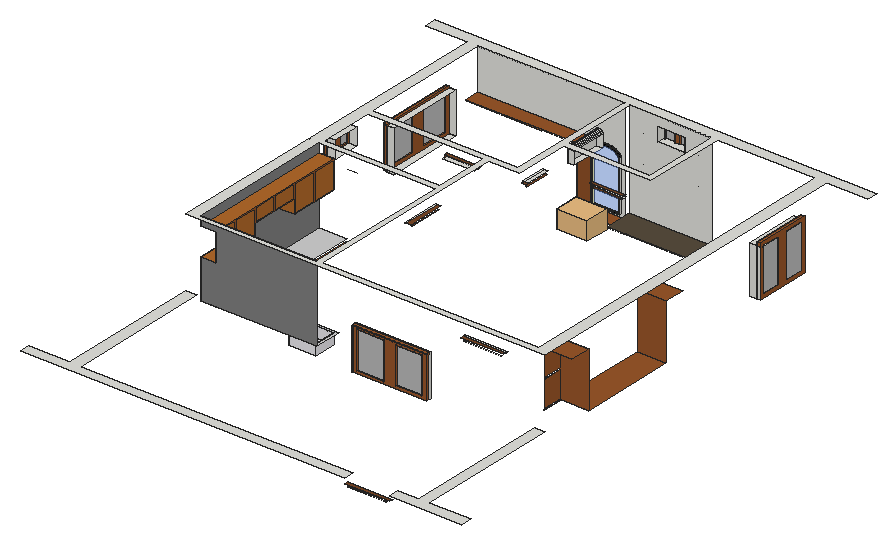
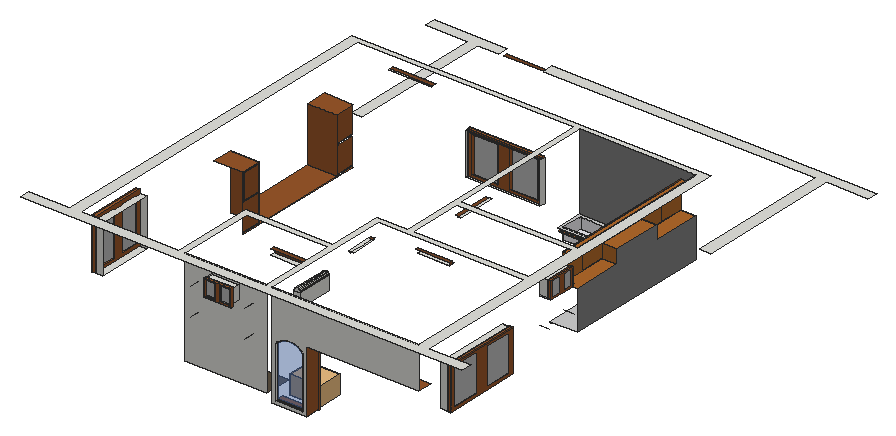
# SketchUp Ruby script. Lengths in inches.
U = 1.inch
M = Sketchup.active_model
def pt(a) = Geom::Point3d.new(a.map { |v| v * U })
def face(e, loops, mat)
  f = e.add_face(loops[0].map { |a| pt(a) })
  loops[1..].each { |l| e.add_face(l.map { |a| pt(a) }).erase! }
  f.material = f.back_material = mat if mat
  f
end
# faces: each face lists its corners as indices into pts; further lists are holes
def faces(e, pts, list, mat = nil) = list.each { |f| face(e, (f[0].is_a?(Array) ? f : [f]).map { |l| l.map { |i| pts[i] } }, mat) }
# xy, xz, yz: faces in a plane at the given z, y or x. An outline is a flat list of corners, or four numbers for a rectangle; further outlines are holes
def ring(l) = l.size == 4 ? [[l[0], l[1]], [l[2], l[1]], [l[2], l[3]], [l[0], l[3]]] : l.each_slice(2).to_a
def flat(e, list, mat, &to3) = list.each { |f| face(e, (f[0].is_a?(Array) ? f : [f]).map { |l| ring(l).map { |u, v| to3.(u, v) } }, mat) }
def xy(e, z, list, mat = nil) = flat(e, list, mat) { |x, y| [x, y, z] }
def xz(e, y, list, mat = nil) = flat(e, list, mat) { |x, z| [x, y, z] }
def yz(e, x, list, mat = nil) = flat(e, list, mat) { |y, z| [x, y, z] }
def lines(e, pts, list) = list.each { |a, b| e.add_line(pt(pts[a]), pt(pts[b])) }
# prism: a flat outline (further loops are holes) pulled along v
def prism(e, loops, v, mat = nil)
  f = face(e, loops, mat); d = Geom::Vector3d.new(v.map { |x| x * U })
  f.pushpull(f.normal.samedirection?(d) ? d.length : -d.length)
end
def box(e, o, s, mat = nil) = prism(e, [[o, [o[0] + s[0], o[1], o[2]], [o[0] + s[0], o[1] + s[1], o[2]], [o[0], o[1] + s[1], o[2]]]], [0, 0, s[2]], mat)
def at(x, y, z, deg = 0) = Geom::Transformation.translation(pt([x, y, z])) * Geom::Transformation.rotation(ORIGIN, Z_AXIS, deg.degrees)
def axes(o, x, y, z) = Geom::Transformation.new([*x, 0, *y, 0, *z, 0, *pt(o).to_a, 1])
def part(name) = M.definitions.add(name)
# library, detail: a bought-in or finely detailed component or shape, given as its bounding box
def library(name, o, s) = part(name).tap { |d| box(d.entities, o, s) }
def detail(e, o, s) = box(e.add_group.entities, o, s)
def put(e, d, t, mat = nil) = e.add_instance(d, t).tap { |i| i.material = mat if mat }
def group(e, t, mat = nil) = e.add_group.tap { |g| g.transformation = t; g.material = mat if mat }.entities
root = M.entities
M.materials.add("[0133_Gray]").color = [128, 128, 128]
M.materials.add("[Carpet Diamond Olive]").color = [87, 77, 61]
M.materials.add("[Carrera Marble]").color = [207, 207, 207]
M.materials.add("[Color E01]").color = [255, 255, 204]
M.materials.add("[Color M09]").color = [0, 0, 0]
M.materials.add("[Metal Silver]").color = [234, 233, 238]
M.materials.add("[Mirror 01]").color = [185, 185, 185]
M.materials.add("[Translucent Glass Blue]").color = [100, 149, 237]
M.materials["[Translucent Glass Blue]"].alpha = 0.5
M.materials.add("[Wood Bamboo]").color = [177, 105, 43]
M.materials.add("[Wood Cherry Original]").color = [152, 86, 42]
M.materials.add("[Wood Veneer 01]").color = [120, 70, 37]
xy(root,40.7,[[157.82,411.42,158.26,411.48,158.67,411.64,159.02,411.87,159.28,412.16,159.43,412.49,159.47,412.85,159.39,413.2,159.19,413.52,158.9,413.79,158.53,413.99,158.1,414.11,157.65,414.14,157.21,414.08,156.8,413.93,156.45,413.7,156.2,413.41,156.04,413.07,156,412.72,156.08,412.37,156.28,412.05,156.57,411.77,156.94,411.57,157.37,411.45]])
xy(root,41.76,[[142.67,429.03,172.1875,429.09]],"[Wood Cherry Original]")
xy(root,42,[[142.43,429.03,172.43,441.09]],"[Wood Cherry Original]")
xy(root,44.5,[[145.43,439.34,169.43,441.09]],"[Color M09]")
xy(root,45.45,[[146.38,439.34,168.48,439.84]],"[Color E01]")
xy(root,47.48,[[177.45,416.84,191.41,417.09]],"[Wood Cherry Original]")
xy(root,47.52,[[234.125,416.84,248.17,417.09]],"[Wood Cherry Original]")
xy(root,47.61,[[192.32,416.84,233.26,417.09]],"[Wood Cherry Original]")
xy(root,48,[[176.93,416.84,248.65,441.09]],"[Carpet Diamond Olive]")
xy(root,56.5,[[[119.52,142.1,143.52,161.1],[131.48,150.16,131.11,150.21,130.76,150.35,130.46,150.58,130.23,150.875,130.09,151.22,130.04,151.6,130.09,151.97,130.23,152.3125,130.46,152.61,130.76,152.84,131.11,152.98,131.48,153.03,131.85,152.98,132.2,152.84,132.5,152.61,132.72,152.3125,132.87,151.97,132.92,151.6,132.87,151.22,132.72,150.875,132.5,150.58,132.2,150.35,131.85,150.21]]],"[Metal Silver]")
xy(root,59.14,[[314.375,278.46,315,294.73]],"[Wood Cherry Original]")
xy(root,59.25,[[314.375,194.35,315,276.84]],"[Wood Cherry Original]")
xy(root,59.27,[[314.375,176.32,315,192.87]],"[Wood Cherry Original]")
xy(root,60,[[180.52,135.1,180.65,135.1,180.65,138.1,244.97,138.1,244.97,139.6,180.52,139.6]])
xy(root,60,[[180.65,135.1,244.97,138.1],[314.375,193.6,339,277.6]],"[Wood Cherry Original]")
xy(root,60.61,[[314.375,278.2,315,294.99]],"[Wood Cherry Original]")
xy(root,60.84,[[314.375,176.44,315,192.76]],"[Wood Cherry Original]")
xy(root,62.06,[[184.23,135.1,207.89,136.6],[184.23,136.6,207.89,138.1]],"[Wood Cherry Original]")
xy(root,62.35,[[218.23,135.1,240.89,136.6],[218.23,136.6,240.89,138.1]],"[Wood Cherry Original]")
xy(root,63.54,[[97.27,163.6,119.56,164.6]],"[Wood Cherry Original]")
xy(root,63.58,[[121.23,163.6,143.6,164.6]],"[Wood Cherry Original]")
xy(root,63.69,[[69,243.75,70,266.29]],"[Wood Cherry Original]")
xy(root,63.7,[[71.3,163.6,95.72,164.6]],"[Wood Cherry Original]")
xy(root,63.76,[[69,217.84,70,242.35]],"[Wood Cherry Original]")
xy(root,63.875,[[69,189.72,70,216.62]],"[Wood Cherry Original]")
xy(root,63.89,[[69,165.7,70,188.63]],"[Wood Cherry Original]")
xy(root,64.4,[[70.6,163.6,144.41,164.6]],"[Wood Cherry Original]")
xy(root,64.43,[[69,165.17,70,267.02]],"[Wood Cherry Original]")
xy(root,66,[[[45,139.6,146.02,139.6,146.02,163.6,69,163.6,69,268.59,45,268.59],[119.52,142.1,143.52,161.1]]],"[Carrera Marble]")
xy(root,66.58,[[284.37,0,318.52,0.61]],"[Wood Veneer 01]")
xy(root,67.92,[[281.85,0,321.03,3.06]],"[Wood Veneer 01]")
xy(root,72,[[0,0.09,281.85,0.09,281.85,9.09,45,9.09,45,135.1,36,135.1,36,9.09,0,9.09],[321.12,0.09,384,0.09,384,9.09,348,9.09,348,135.1,339,135.1,339,9.09,321.12,9.09],[36,349.59,39,417.09],[39,349.59,45,417.09],[339,369.09,344.8125,417.09]])
xy(root,72,[[344.8125,369.09,348,417.09],[36,417.09,39,417.39]],"[Wood Cherry Original]")
xy(root,74.05,[[36,388.68,37.5,413.62],[37.5,388.68,39,413.62]],"[Wood Cherry Original]")
xy(root,74.34,[[36,353.9,37.5,377.78],[37.5,353.9,39,377.78]],"[Wood Cherry Original]")
xy(root,74.46,[[344.8125,396.76,346.5,414.42],[346.5,396.76,348,414.42]],"[Wood Cherry Original]")
xy(root,74.8,[[344.8125,372.14,346.5,389.05],[346.5,372.14,348,389.05]],"[Wood Cherry Original]")
xy(root,83.16,[[314.375,176.44,315,192.76]],"[Wood Cherry Original]")
xy(root,83.39,[[314.375,278.2,315,294.99]],"[Wood Cherry Original]")
xy(root,84.87,[[314.375,176.47,315,192.73]],"[Wood Cherry Original]")
xy(root,84.9,[[314.375,278.49,315,294.7]],"[Wood Cherry Original]")
xy(root,94.61,[[218.23,135.1,240.89,136.6],[218.23,136.6,240.89,138.1]],"[Wood Cherry Original]")
xy(root,94.9,[[184.23,135.1,207.89,136.6],[184.23,136.6,207.89,138.1]],"[Wood Cherry Original]")
xy(root,95,[[76,427.9,111.43,429.09]],"[Wood Cherry Original]")
xy(root,95.11,[[45.89,427.9,74.11,429.09]],"[Wood Cherry Original]")
xy(root,95.125,[[113.31,427.9,141.56,429.09]],"[Wood Cherry Original]")
xy(root,96,[[180.52,135.1,244.97,139.6]])
xy(root,96,[[45,427.9,142.43,441.09]],"[Wood Cherry Original]")
xy(root,96.96,[[180.65,135.1,244.97,138.1]],"[Wood Cherry Original]")
xy(root,100,[[45,139.6,58,182.8],[45,225.39,58,268.59]],"[Wood Bamboo]")
xy(root,100.29,[[57.6875,225.68,58,246.7]],"[Wood Cherry Original]")
xy(root,100.3,[[57.6875,247.29,58,268.29]],"[Wood Cherry Original]")
xy(root,100.52,[[57.6875,161.71,58,182.28]],"[Wood Cherry Original]")
xy(root,100.57,[[57.6875,140.16,58,160.63]],"[Wood Cherry Original]")
xy(root,106.46,[[36,353.9,37.5,377.78],[37.5,353.9,39,377.78]],"[Wood Cherry Original]")
xy(root,106.75,[[36,388.68,37.5,413.62],[37.5,388.68,39,413.62]],"[Wood Cherry Original]")
xy(root,107.1,[[314.375,278.49,315,294.7]],"[Wood Cherry Original]")
xy(root,107.13,[[314.375,176.47,315,192.73]],"[Wood Cherry Original]")
xy(root,107.625,[[166.49,386.4,172.43,417.09]])
xy(root,108,[[36,349.59,45,417.09],[200.53,369.09,227.35,373.59]])
xy(root,108,[[314.375,175.6,339,193.6],[314.375,277.6,339,295.6]],"[Wood Cherry Original]")
xy(root,108.8,[[36,349.59,39,417.39]],"[Wood Cherry Original]")
xy(root,109.55,[[202.14,368.53,227.35,369.09]],"[Wood Veneer 01]")
xy(root,110.07,[[200.77,447.84,200.85,450.09],[200.85,447.84,224.85,450.09]],"[Wood Cherry Original]")
xy(root,110.9,[[214.65,447.84,223.51,448.97],[214.65,448.97,223.51,450.09]],"[Wood Cherry Original]")
xy(root,111.02,[[202.3,447.84,210.78,448.97],[202.3,448.97,210.78,450.09]],"[Wood Cherry Original]")
xy(root,111.53,[[200.28,368.53,229.21,371.34]],"[Wood Veneer 01]")
xy(root,112,[[36,285.01,36,285.09,45,285.09,45,309.09,38.25,309.09,38.25,285.01],[200.93,441.09,224.65,450.09]])
xy(root,112,[[45,182.8,58,225.39]],"[Wood Bamboo]")
xy(root,112,[[36,285.01,38.25,285.09],[36,285.09,38.25,309.09]],"[Wood Cherry Original]")
xy(root,112.19,[[57.6875,183.15,58,203.39],[57.6875,203.93,58,225.2]],"[Wood Cherry Original]")
xy(root,112.83,[[36,298.89,37.125,307.75],[37.125,298.89,38.25,307.75]],"[Wood Cherry Original]")
xy(root,112.95,[[36,286.54,37.125,295.02],[37.125,286.54,38.25,295.02]],"[Wood Cherry Original]")
xy(root,113,[[339,369.09,348,417.09]])
xy(root,113.36,[[344.8125,372.14,346.5,389.05],[346.5,372.14,348,389.05]],"[Wood Cherry Original]")
xy(root,113.7,[[344.8125,396.76,346.5,414.42],[346.5,396.76,348,414.42]],"[Wood Cherry Original]")
xy(root,116.16,[[344.8125,369.09,348,417.09]],"[Wood Cherry Original]")
xy(root,117.89,[[277.36,135.1,309.79,135.66],[149.95,237.83,150.52,266.48],[176.37,329.24,176.93,350.51]],"[Wood Veneer 01]")
xy(root,118.9375,[[166.49,386.4,166.52,417.09],[172.4,386.4,172.43,417.09]])
xy(root,120,[[274.97,137.91,312.18,139.6],[146.02,235.72,147.7,268.59],[110.58,321.09,137.86,325.59],[172.43,330.47,174.12,352.08],[174.12,330.47,176.93,352.08]])
xy(root,120,[[274.97,135.1,312.18,137.91],[147.7,235.72,150.52,268.59],[112.49,325.03,138.36,325.59],[174.12,327.67,176.93,330.47]],"[Wood Veneer 01]")
xy(root,122.16,[[110.58,322.78,140.27,325.59]],"[Wood Veneer 01]")
xy(root,123.43,[[57.6875,140.16,58,160.63]],"[Wood Cherry Original]")
xy(root,123.48,[[57.6875,161.71,58,182.28]],"[Wood Cherry Original]")
xy(root,123.65,[[57.6875,183.15,58,203.39]],"[Wood Cherry Original]")
xy(root,123.7,[[57.6875,247.29,58,268.29]],"[Wood Cherry Original]")
xy(root,123.71,[[57.6875,225.68,58,246.7]],"[Wood Cherry Original]")
xy(root,123.81,[[57.6875,203.93,58,225.2]],"[Wood Cherry Original]")
xy(root,124,[[200.93,441.09,224.65,450.09]])
xy(root,124,[[45,139.6,58,268.59]],"[Wood Bamboo]")
xy(root,124.11,[[202.3,447.84,210.78,448.97],[202.3,448.97,210.78,450.09]],"[Wood Cherry Original]")
xy(root,124.23,[[214.65,447.84,223.51,448.97],[214.65,448.97,223.51,450.09]],"[Wood Cherry Original]")
xy(root,125.07,[[200.77,447.84,200.85,450.09],[200.85,447.84,224.85,450.09]],"[Wood Cherry Original]")
xy(root,126.05,[[36,286.54,37.125,295.02],[37.125,286.54,38.25,295.02]],"[Wood Cherry Original]")
xy(root,126.17,[[36,298.89,37.125,307.75],[37.125,298.89,38.25,307.75]],"[Wood Cherry Original]")
xy(root,127,[[36,285.01,38.25,285.01,38.25,309.09,45,309.09,45,285.09,36,285.09]])
xy(root,127,[[36,285.01,38.25,285.09],[36,285.09,38.25,309.09]],"[Wood Cherry Original]")
xy(root,132,[[[36,135.1,348,135.1,348,441.09,384,441.09,384,450.09,0,450.09,0,441.09,36,441.09,36,268.59,146.02,268.59,146.02,139.6,45,139.6,45,268.59,36,268.59],[150.52,139.6,150.52,321.09,176.93,321.09,176.93,369.09,253.15,369.09,253.15,441.09,339,441.09,339,139.6],[45,325.59,172.43,441.09],[45,273.09,146.02,321.09],[176.93,373.59,248.65,441.09]]])
xz(root,135.1,[[[180.65,60,244.97,96],[184.23,62.06,207.89,94.9],[218.23,62.35,240.89,94.61]],[180.65,96,244.97,96.96]],"[Wood Cherry Original]")
xz(root,136.6,[[184.23,62.06,207.89,94.9],[218.23,62.35,240.89,94.61]],"[Mirror 01]")
xz(root,138.1,[[[180.65,60,244.97,96.96],[184.23,62.06,207.89,94.9],[218.23,62.35,240.89,94.61]]],"[Wood Cherry Original]")
xz(root,139.6,[[45,66,45,100,58,100,58,124,45,124,45,132,146.02,132,146.02,66]],"[0133_Gray]")
xz(root,140.16,[[57.6875,100.57,58,123.43]],"[Wood Cherry Original]")
xz(root,142.1,[[119.52,56.5,143.52,66]],"[Metal Silver]")
xz(root,160.63,[[57.6875,100.57,58,123.43]],"[Wood Cherry Original]")
xz(root,161.1,[[119.52,56.5,143.52,66]],"[Metal Silver]")
xz(root,161.71,[[57.6875,100.52,58,123.48]],"[Wood Cherry Original]")
xz(root,176.44,[[314.375,60.84,315,83.16]],"[Wood Cherry Original]")
xz(root,176.47,[[314.375,84.87,315,107.13]],"[Wood Cherry Original]")
xz(root,182.28,[[57.6875,100.52,58,112],[57.6875,112,58,123.48]],"[Wood Cherry Original]")
xz(root,182.8,[[45,100,58,112]],"[Wood Bamboo]")
xz(root,183.15,[[57.6875,112.19,58,112.35]])
xz(root,183.15,[[57.6875,112.35,58,123.65]],"[Wood Cherry Original]")
xz(root,192.73,[[314.375,84.87,315,107.13]],"[Wood Cherry Original]")
xz(root,192.76,[[314.375,60.84,315,83.16]],"[Wood Cherry Original]")
xz(root,193.6,[[314.375,60,339,108]],"[Wood Cherry Original]")
xz(root,203.39,[[57.6875,112.19,58,112.35],[57.6875,112.35,58,123.65]],"[Wood Cherry Original]")
xz(root,203.93,[[57.6875,112.19,58,123.81]],"[Wood Cherry Original]")
xz(root,225.2,[[57.6875,112.19,58,123.81]],"[Wood Cherry Original]")
xz(root,225.39,[[45,100,58,112]],"[Wood Bamboo]")
xz(root,225.68,[[57.6875,100.29,58,112],[57.6875,112,58,123.71]],"[Wood Cherry Original]")
xz(root,246.7,[[57.6875,100.29,58,123.71]],"[Wood Cherry Original]")
xz(root,247.29,[[57.6875,100.3,58,123.7]],"[Wood Cherry Original]")
xz(root,268.29,[[57.6875,100.3,58,123.7]],"[Wood Cherry Original]")
xz(root,277.6,[[314.375,60,339,108]],"[Wood Cherry Original]")
xz(root,278.2,[[314.375,60.61,315,83.39]],"[Wood Cherry Original]")
xz(root,278.49,[[314.375,84.9,315,107.1]],"[Wood Cherry Original]")
xz(root,285.01,[[36,112,38.25,127]],"[Wood Cherry Original]")
xz(root,285.09,[[36,112,45,127]])
xz(root,286.54,[[36,112.95,37.125,126.05],[37.125,112.95,38.25,126.05]],"[Wood Cherry Original]")
xz(root,294.7,[[314.375,84.9,315,107.1]],"[Wood Cherry Original]")
xz(root,294.99,[[314.375,60.61,315,83.39]],"[Wood Cherry Original]")
xz(root,295.02,[[36,112.95,37.125,126.05],[37.125,112.95,38.25,126.05]],"[Wood Cherry Original]")
xz(root,298.89,[[36,112.83,37.125,126.17],[37.125,112.83,38.25,126.17]],"[Wood Cherry Original]")
xz(root,307.75,[[36,112.83,37.125,126.17],[37.125,112.83,38.25,126.17]],"[Wood Cherry Original]")
xz(root,309.09,[[38.25,112,45,127]])
xz(root,309.09,[[36,112,38.25,127]],"[Wood Cherry Original]")
xz(root,349.59,[[39,72,45,108]])
xz(root,349.59,[[36,72,39,108],[36,108,39,108.8]],"[Wood Cherry Original]")
xz(root,353.9,[[36,74.34,37.5,106.46],[37.5,74.34,39,106.46]],"[Wood Cherry Original]")
xz(root,369.09,[[339,72,344.8125,113],[344.8125,72,348,113]])
xz(root,369.09,[[344.8125,113,348,116.16]],"[Wood Cherry Original]")
xz(root,369.09,[[202.14,108,227.35,109.55]],"[Wood Veneer 01]")
xz(root,372.14,[[344.8125,74.8,346.5,113.36],[346.5,74.8,348,113.36]],"[Wood Cherry Original]")
xz(root,377.78,[[36,74.34,37.5,106.46],[37.5,74.34,39,106.46]],"[Wood Cherry Original]")
xz(root,386.4,[[166.49,107.625,172.43,118.9375],[166.52,118.9375,172.4,118.9375,172.3,119.7,172.01,120.41,171.54,121.01,170.93,121.48,170.22,121.77,169.46,121.875,168.7,121.77,167.99,121.48,167.38,121.01,166.92,120.41,166.625,119.7]])
xz(root,388.68,[[36,74.05,37.5,106.75],[37.5,74.05,39,106.75]],"[Wood Cherry Original]")
xz(root,389.05,[[344.8125,74.8,346.5,113.36],[346.5,74.8,348,113.36]],"[Wood Cherry Original]")
xz(root,396.76,[[344.8125,74.46,346.5,113.7],[346.5,74.46,348,113.7]],"[Wood Cherry Original]")
xz(root,413.62,[[36,74.05,37.5,106.75],[37.5,74.05,39,106.75]],"[Wood Cherry Original]")
xz(root,414.42,[[344.8125,74.46,346.5,113.7],[346.5,74.46,348,113.7]],"[Wood Cherry Original]")
xz(root,417.09,[[36,72,45,108],[339,72,344.8125,113],[166.49,107.625,172.43,118.9375],[166.52,118.9375,166.625,119.7,166.92,120.41,167.38,121.01,167.99,121.48,168.7,121.77,169.46,121.875,170.22,121.77,170.93,121.48,171.54,121.01,172.01,120.41,172.3,119.7,172.4,118.9375]])
xz(root,417.09,[[344.8125,72,348,113],[344.8125,113,348,116.16]],"[Wood Cherry Original]")
xz(root,417.39,[[36,72,39,108.8]],"[Wood Cherry Original]")
xz(root,439.34,[[[145.43,44.5,169.43,44.5,169.43,89.29,168.04,91.11,164.93,93.49,161.3125,94.99,157.43,95.5,153.55,94.99,149.93,93.49,146.82,91.11,145.43,89.29],[146.38,45.45,146.38,88.97,147.5,90.43,150.41,92.66,153.8,94.0625,157.43,94.54,161.06,94.0625,164.45,92.66,167.36,90.43,168.48,88.97,168.48,45.45]]],"[Color M09]")
xz(root,439.84,[[146.38,45.45,168.48,45.45,168.48,88.97,167.36,90.43,164.45,92.66,161.06,94.0625,157.43,94.54,153.8,94.0625,150.41,92.66,147.5,90.43,146.38,88.97]],"[Translucent Glass Blue]")
xz(root,441.09,[[[142.43,42,172.43,42,172.43,132,45,132,45,96,142.43,96],[145.43,44.5,145.43,89.29,146.82,91.11,149.93,93.49,153.55,94.99,157.43,95.5,161.3125,94.99,164.93,93.49,168.04,91.11,169.43,89.29,169.43,44.5]],[[176.93,48,248.65,132],[200.93,112,224.65,124]]])
xz(root,447.84,[[[200.77,110.07,224.85,125.07],[214.65,110.9,223.51,124.23],[202.3,111.02,210.78,124.11]]],"[Wood Cherry Original]")
xz(root,448.97,[[214.65,110.9,223.51,124.23],[202.3,111.02,210.78,124.11]],"[Mirror 01]")
xz(root,450.09,[[200.77,110.07,200.85,125.07],[[200.85,110.07,224.85,125.07],[214.65,110.9,223.51,124.23],[202.3,111.02,210.78,124.11]]],"[Wood Cherry Original]")
yz(root,36,[[417.09,72,417.09,108,349.59,108,349.59,108.8,417.39,108.8,417.39,72],[[349.59,72,417.09,108],[388.68,74.05,413.62,106.75],[353.9,74.34,377.78,106.46]],[285.01,112,285.09,127],[[285.09,112,309.09,127],[298.89,112.83,307.75,126.17],[286.54,112.95,295.02,126.05]]],"[Wood Cherry Original]")
yz(root,37.125,[[298.89,112.83,307.75,126.17],[286.54,112.95,295.02,126.05]],"[Mirror 01]")
yz(root,37.5,[[388.68,74.05,413.62,106.75],[353.9,74.34,377.78,106.46]],"[Mirror 01]")
yz(root,38.25,[[[285.01,112,309.09,127],[298.89,112.83,307.75,126.17],[286.54,112.95,295.02,126.05]]],"[Wood Cherry Original]")
yz(root,39,[[[349.59,72,417.39,108.8],[388.68,74.05,413.62,106.75],[353.9,74.34,377.78,106.46]]],"[Wood Cherry Original]")
yz(root,45,[[139.6,66,268.59,66,268.59,100,225.39,100,225.39,112,182.8,112,182.8,100,139.6,100],[139.6,124,268.59,132]],"[0133_Gray]")
yz(root,57.6875,[[225.68,100.29,246.7,123.71],[247.29,100.3,268.29,123.7],[161.71,100.52,182.28,123.48],[140.16,100.57,160.63,123.43],[183.15,112.19,203.39,123.65],
  [203.93,112.19,225.2,123.81]],"[Wood Bamboo]")
yz(root,58,[[[139.6,100,182.8,100,182.8,112,225.39,112,225.39,100,268.59,100,268.59,124,139.6,124],[225.68,100.29,246.7,123.71],[247.29,100.3,268.29,123.7],[161.71,100.52,182.28,123.48],[140.16,100.57,160.63,123.43],[203.93,112.19,225.2,123.81],[183.15,112.19,203.39,123.65]]],"[Wood Cherry Original]")
yz(root,110.58,[[322.78,120,325.59,122.16]],"[Wood Veneer 01]")
yz(root,119.52,[[142.1,56.5,161.1,66]],"[Metal Silver]")
yz(root,141.56,[[427.9,42,429.09,95.125]],"[Wood Cherry Original]")
yz(root,142.43,[[427.9,42,441.09,96]],"[Wood Cherry Original]")
yz(root,143.52,[[142.1,56.5,161.1,66]],"[Metal Silver]")
yz(root,145.43,[[439.34,44.5,441.09,89.29]],"[Color M09]")
yz(root,146.38,[[439.34,45.45,439.84,88.97]],"[Color E01]")
yz(root,166.49,[[386.4,107.625,417.09,118.9375]])
yz(root,168.48,[[439.34,45.45,439.84,88.97]],"[Color E01]")
yz(root,169.43,[[439.34,44.5,441.09,89.29]])
yz(root,180.52,[[135.1,60,139.6,96]])
yz(root,180.65,[[135.1,60,138.1,96.96]],"[Wood Cherry Original]")
yz(root,184.23,[[135.1,62.06,136.6,94.9],[136.6,62.06,138.1,94.9]],"[Wood Cherry Original]")
yz(root,200.77,[[447.84,110.07,450.09,125.07]],"[Wood Cherry Original]")
yz(root,200.93,[[441.09,112,450.09,124]])
yz(root,202.3,[[447.84,111.02,448.97,124.11],[448.97,111.02,450.09,124.11]],"[Wood Cherry Original]")
yz(root,207.89,[[135.1,62.06,136.6,94.9],[136.6,62.06,138.1,94.9]],"[Wood Cherry Original]")
yz(root,210.78,[[447.84,111.02,448.97,124.11],[448.97,111.02,450.09,124.11]],"[Wood Cherry Original]")
yz(root,214.65,[[447.84,110.9,448.97,124.23],[448.97,110.9,450.09,124.23]],"[Wood Cherry Original]")
yz(root,218.23,[[135.1,62.35,136.6,94.61],[136.6,62.35,138.1,94.61]],"[Wood Cherry Original]")
yz(root,223.51,[[447.84,110.9,448.97,124.23],[448.97,110.9,450.09,124.23]],"[Wood Cherry Original]")
yz(root,224.65,[[441.09,112,450.09,124]])
yz(root,224.85,[[447.84,110.07,450.09,125.07]],"[Wood Cherry Original]")
yz(root,240.89,[[135.1,62.35,136.6,94.61],[136.6,62.35,138.1,94.61]],"[Wood Cherry Original]")
yz(root,244.97,[[138.1,60,139.6,96]])
yz(root,244.97,[[135.1,60,138.1,96],[135.1,96,138.1,96.96]],"[Wood Cherry Original]")
yz(root,315,[[278.2,60.61,294.99,83.39],[176.44,60.84,192.76,83.16],[176.47,84.87,192.73,107.13],[278.49,84.9,294.7,107.1]],"[Wood Cherry Original]")
yz(root,344.8125,[[[369.09,72,417.09,116.16],[396.76,74.46,414.42,113.7],[372.14,74.8,389.05,113.36]]],"[Wood Cherry Original]")
yz(root,346.5,[[396.76,74.46,414.42,113.7],[372.14,74.8,389.05,113.36]],"[Mirror 01]")
yz(root,348,[[[369.09,72,417.09,116.16],[396.76,74.46,414.42,113.7],[372.14,74.8,389.05,113.36]]],"[Wood Cherry Original]")
p = [[147.5,439.34,90.43],[146.38,439.34,88.97],[146.38,439.84,88.97],[147.5,439.84,90.43],[168.48,439.34,88.97],[167.36,439.34,90.43],
  [167.36,439.84,90.43],[168.48,439.84,88.97],[146.82,441.09,91.11],[145.43,441.09,89.29],[145.43,439.34,89.29],[146.82,439.34,91.11],
  [169.43,441.09,89.29],[168.04,441.09,91.11],[168.04,439.34,91.11],[169.43,439.34,89.29],[150.41,439.34,92.66],[150.41,439.84,92.66],
  [164.45,439.34,92.66],[164.45,439.84,92.66],[149.93,441.09,93.49],[149.93,439.34,93.49],[164.93,441.09,93.49],[164.93,439.34,93.49],
  [153.8,439.34,94.0625],[153.8,439.84,94.0625],[161.06,439.34,94.0625],[161.06,439.84,94.0625],[153.55,441.09,94.99],[153.55,439.34,94.99],
  [161.3125,441.09,94.99],[161.3125,439.34,94.99],[157.43,439.34,94.54],[157.43,439.84,94.54],[157.43,441.09,95.5],[157.43,439.34,95.5],
  [166.52,386.4,118.9375],[166.625,386.4,119.7],[166.625,417.09,119.7],[166.52,417.09,118.9375],[172.3,386.4,119.7],[172.4,386.4,118.9375],
  [172.4,417.09,118.9375],[172.3,417.09,119.7],[166.92,386.4,120.41],[166.92,417.09,120.41],[172.01,386.4,120.41],[172.01,417.09,120.41],
  [167.38,386.4,121.01],[167.38,417.09,121.01],[171.54,386.4,121.01],[171.54,417.09,121.01],[167.99,386.4,121.48],[167.99,417.09,121.48],
  [170.93,386.4,121.48],[170.93,417.09,121.48],[168.7,386.4,121.77],[168.7,417.09,121.77],[170.22,386.4,121.77],[170.22,417.09,121.77],
  [169.46,386.4,121.875],[169.46,417.09,121.875],[236.65,441.09,114],[236.65,450.09,114],[236.65,441.09,90],[236.65,450.09,90],
  [188.93,441.09,114],[188.93,450.09,114],[188.93,441.09,90],[188.93,450.09,90],[45,283.4,114],[36,283.4,114],
  [45,310.4,114],[36,310.4,114],[45,283.4,90],[36,283.4,90],[45,310.4,90],[36,310.4,90],
  [169.46,386.4,121.9375]]
faces(root,p,[[0,1,2,3],[4,5,6,7],[16,0,3,17],[5,18,19,6],[24,16,17,25],[18,26,27,19],[32,24,25,33],[26,32,33,27]],"[Color E01]")
faces(root,p,[[8,9,10,11],[12,13,14,15],[20,8,11,21],[13,22,23,14],[28,20,21,29],[22,30,31,23],[34,28,29,35],[30,34,35,31]],"[Color M09]")
faces(root,p,[[36,37,38,39],[40,41,42,43],[37,44,45,38],[46,40,43,47],[44,48,49,45],[50,46,47,51],[48,52,53,49],[54,50,51,55],
  [52,56,57,53],[58,54,55,59],[56,60,61,57],[60,58,59,61]])
lines(root,p,[[62,63],[64,65],[66,67],[68,69],[70,71],[72,73],[74,75],[76,77],[60,78]])
detail(root,[144.48,402.36,41.11],[26.51,20.87,16.16])
